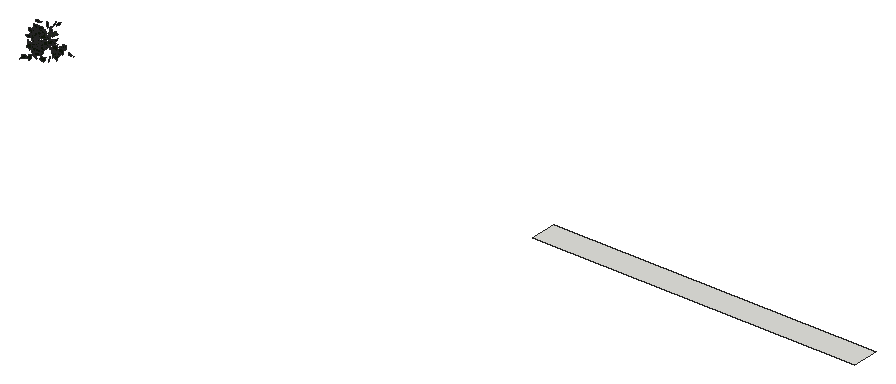
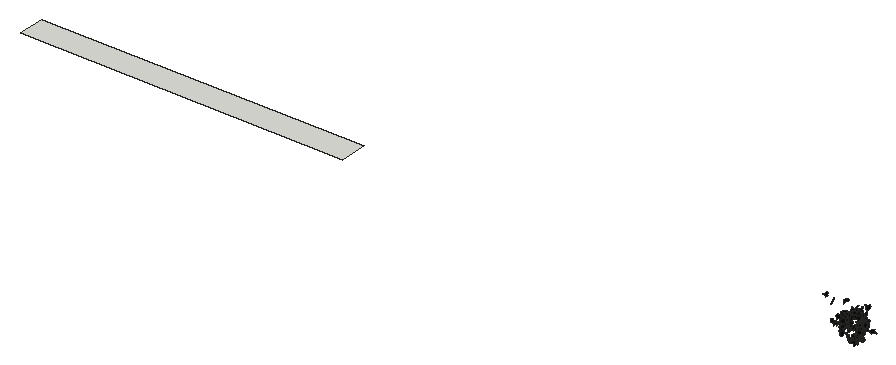
# SketchUp Ruby script. Lengths in inches.
U = 1.inch
M = Sketchup.active_model
def pt(a) = Geom::Point3d.new(a.map { |v| v * U })
def face(e, loops, mat)
  f = e.add_face(loops[0].map { |a| pt(a) })
  loops[1..].each { |l| e.add_face(l.map { |a| pt(a) }).erase! }
  f.material = f.back_material = mat if mat
  f
end
# faces: each face lists its corners as indices into pts; further lists are holes
def faces(e, pts, list, mat = nil) = list.each { |f| face(e, (f[0].is_a?(Array) ? f : [f]).map { |l| l.map { |i| pts[i] } }, mat) }
# xy, xz, yz: faces in a plane at the given z, y or x. An outline is a flat list of corners, or four numbers for a rectangle; further outlines are holes
def ring(l) = l.size == 4 ? [[l[0], l[1]], [l[2], l[1]], [l[2], l[3]], [l[0], l[3]]] : l.each_slice(2).to_a
def flat(e, list, mat, &to3) = list.each { |f| face(e, (f[0].is_a?(Array) ? f : [f]).map { |l| ring(l).map { |u, v| to3.(u, v) } }, mat) }
def xy(e, z, list, mat = nil) = flat(e, list, mat) { |x, y| [x, y, z] }
def xz(e, y, list, mat = nil) = flat(e, list, mat) { |x, z| [x, y, z] }
def yz(e, x, list, mat = nil) = flat(e, list, mat) { |y, z| [x, y, z] }
def lines(e, pts, list) = list.each { |a, b| e.add_line(pt(pts[a]), pt(pts[b])) }
# prism: a flat outline (further loops are holes) pulled along v
def prism(e, loops, v, mat = nil)
  f = face(e, loops, mat); d = Geom::Vector3d.new(v.map { |x| x * U })
  f.pushpull(f.normal.samedirection?(d) ? d.length : -d.length)
end
def box(e, o, s, mat = nil) = prism(e, [[o, [o[0] + s[0], o[1], o[2]], [o[0] + s[0], o[1] + s[1], o[2]], [o[0], o[1] + s[1], o[2]]]], [0, 0, s[2]], mat)
def at(x, y, z, deg = 0) = Geom::Transformation.translation(pt([x, y, z])) * Geom::Transformation.rotation(ORIGIN, Z_AXIS, deg.degrees)
def axes(o, x, y, z) = Geom::Transformation.new([*x, 0, *y, 0, *z, 0, *pt(o).to_a, 1])
def part(name) = M.definitions.add(name)
# library, detail: a bought-in or finely detailed component or shape, given as its bounding box
def library(name, o, s) = part(name).tap { |d| box(d.entities, o, s) }
def detail(e, o, s) = box(e.add_group.entities, o, s)
def put(e, d, t, mat = nil) = e.add_instance(d, t).tap { |i| i.material = mat if mat }
def group(e, t, mat = nil) = e.add_group.tap { |g| g.transformation = t; g.material = mat if mat }.entities
root = M.entities
M.materials.add("efeu1").color = [18, 25, 13]
M.materials.add("efeu2").color = [43, 57, 29]
c1 = part("ivyleaf_10")
p = [[0,0.5,-0.03],[-0.0625,2.02,-0.43],[-0.19,2.01,-0.46],[-0.54,1.05,-0.29],[-0.52,0.625,-0.18],[-0.83,0.76,-0.28],
  [-1.16,0.64,-0.33],[-1.15,0.33,-0.24],[-0.77,-0.39,0.02],[-0.3,-0.51,0.16],[0.04,-0.48,0.23],[-0.02,2.01,-0.4375],
  [-0.06,2.01,-0.43],[0.04,-0.49,0.23],[0.67,-0.49,0.14],[1.38,0.36,-0.2],[1.375,0.51,-0.24],[0.81,0.65,-0.19],
  [0.62,0.59,-0.15],[0.6,1.09,-0.28],[0.5,1.23,-0.31]]
faces(c1.entities,p,[[0,1,2,3,4,5,6,7,8,9,10],[11,12,0,13,14,15,16,17,18,19,20]],"efeu2")
c2 = part("ivyleaf_9")
p = [[1.54,2.16,1.25],[1.36,2.04,1.19],[-0.21,0.99,0.68],[-0.71,1.11,0.82],[-0.85,0.86,0.67],[-0.8,0.17,0.21],
  [-0.9,-0.01,0.1],[-0.67,-0.16,-0.02],[-0.08,-0.08,-0.05],[-0.03,-0.6,-0.4],[0.65,-0.88,-0.66],[0.83,-0.6,-0.49],
  [1.29,-0.42,-0.43],[1.8125,-0.07,-0.26],[1.21,0.44,0.15]]
faces(c2.entities,p,[[0,1,2,3,4,5,6,7,8,9,10,11,12,13,14]],"efeu1")
xy(root,234.35,[[233.9,223.4375,351.16,233.25]])
put(root,c1,axes([53.68,222.76,235.85],[0.26866,-0.3585,-0.22203],[-0.10987,0.19466,-0.44725],[0.40712,0.28911,0.02581]))
put(root,c1,axes([53.39,224.44,234.02],[0.06431,-0.20007,0.45369],[0.33751,-0.31749,-0.18785],[0.36325,0.33041,0.09422]))
put(root,c2,axes([53.25,220.89,238.05],[0.09206,-0.15249,0.4672],[0.48376,-0.05563,-0.11348],[0.08659,0.47292,0.1373]))
put(root,c2,axes([53.3,223.6875,241.74],[0.41396,-0.06275,0.27331],[0.28028,0.10827,-0.39965],[-0.00903,0.48409,0.12482]))
put(root,c2,axes([53.38,223.2,239.45],[0.45441,-0.09026,0.18806],[0.19009,-0.00644,-0.46241],[0.0859,0.49174,0.02846]))
put(root,c2,axes([53.79,222.93,236.93],[0.2925,0.38007,-0.14139],[-0.08119,-0.11592,-0.47955],[-0.39731,0.3035,-0.0061]))
put(root,c1,axes([53.71,222.47,239.98],[0.36999,0.33148,-0.05681],[-0.0427,-0.03749,-0.49676],[-0.33359,0.37245,0.00057]))
put(root,c1,axes([53.66,222.33,238.65],[0.48401,-0.09672,0.07988],[0.0795,-0.00978,-0.49354],[0.09703,0.49046,0.00591]))
put(root,c1,axes([53.44,222.5,240.39],[0.32317,-0.37959,-0.0384],[0.3815,0.32203,0.02744],[0.0039,-0.04703,0.49777]))
put(root,c2,axes([53.7,221.08,240.375],[0.14894,0.13583,0.45757],[0.24086,0.39243,-0.1949],[-0.41207,0.27847,0.05147]))
put(root,c2,axes([53.62,222.21,240.14],[0.24413,-0.42175,-0.11194],[-0.0519,0.0993,-0.48728],[0.43325,0.24954,0.00471]))
put(root,c1,axes([53.51,222.35,241.07],[0.32319,-0.38031,0.03027],[0.38151,0.322,-0.02773],[0.00159,0.04102,0.49831]))
put(root,c2,axes([53.9375,221.61,238.37],[0.22114,-0.11467,-0.43353],[-0.39527,0.17846,-0.24883],[0.2118,0.45277,-0.01173]))
put(root,c1,axes([53.49,221.5625,233.52],[0.06061,-0.08172,0.48954],[0.4629,0.1872,-0.02606],[-0.17902,0.45638,0.09834]))
put(root,c2,axes([53.61,222.13,239.21],[0.48767,-0.1102,-0.00546],[-0.00507,0.00231,-0.49997],[0.11022,0.4877,0.00113]))
put(root,c1,axes([53.97,223.37,234.39],[-0.45789,0.20073,0.00706],[-0.0063,0.0032,-0.49995],[-0.20075,-0.45793,-0.0004]))
put(root,c2,axes([53.83,223.04,237.98],[0.09084,-0.4905,0.03403],[0.00048,-0.03452,-0.49881],[0.49168,0.09065,-0.0058]))
put(root,c2,axes([53.79,220.46,240.29],[0.45416,0.1309,0.16312],[0.15632,0.04662,-0.47264],[-0.13895,0.4803,0.00142]))
put(root,c2,axes([54.3,222.09,237.47],[-0.14055,0.47895,-0.02926],[0.00706,-0.02842,-0.49914],[-0.47979,-0.14072,0.00123]))
put(root,c2,axes([53.87,218.93,236.71],[-0.02657,0.01155,0.49916],[0.20062,-0.45749,0.02126],[0.45722,0.20141,0.01968]))
put(root,c1,axes([54.1,223.16,239.02],[0.49572,-0.06377,-0.01387],[-0.01312,0.00673,-0.49978],[0.06393,0.49587,0.005]))
put(root,c2,axes([54.4375,222.8,239.85],[-0.35492,-0.14761,0.31975],[-0.29035,-0.13428,-0.38427],[0.19932,-0.45845,0.0096]))
put(root,c2,axes([54.45,222.9,239.24],[-0.30345,-0.09684,0.3854],[-0.34664,-0.17261,-0.3163],[0.19431,-0.45916,0.03762]))
put(root,c2,axes([54.48,216.4375,233.95],[-0.04559,0.08062,-0.49135],[-0.06631,-0.48999,-0.07424],[-0.49348,0.05839,0.05536]))
put(root,c2,axes([53.93,221.36,233.76],[0.19913,-0.00962,-0.45854],[0.44578,0.12158,0.19104],[0.10782,-0.4849,0.057]))
put(root,c2,axes([54.51,222.06,239.64],[0.10126,0.48645,-0.05583],[-0.08733,-0.03816,-0.49083],[-0.48179,0.10915,0.07723]))
put(root,c2,axes([54.33,221.63,240.72],[-0.36068,-0.31065,-0.153],[0.18207,0.01779,-0.46533],[0.29456,-0.39138,0.10029]))
put(root,c2,axes([54.17,219.17,236.59],[0.00133,0.00238,-0.49999],[0.49946,-0.02322,0.00122],[-0.02321,-0.49946,-0.00244]))
put(root,c2,axes([54.21,219.32,241.29],[0.25744,-0.4108,0.12233],[0.07922,-0.09464,-0.48453],[0.42125,0.26886,0.01636]))
put(root,c2,axes([54.71,222,240.4],[0.07366,0.47875,0.12397],[-0.04191,0.13093,-0.48073],[-0.49277,0.06043,0.05942]))
put(root,c2,axes([54.68,224.24,234.8125],[-0.21792,-0.23525,0.38363],[-0.18519,-0.3416,-0.31467],[0.41014,-0.27923,0.06175]))
put(root,c2,axes([54.55,221.98,236.875],[0.33559,0.37048,0.01095],[0.00649,0.0089,-0.49988],[-0.37059,0.33565,0.00116]))
put(root,c2,axes([54.79,222.89,234.01],[-0.42098,-0.25223,0.0957],[-0.06874,-0.07121,-0.4901],[0.26087,-0.4258,0.02528]))
put(root,c2,axes([54.25,224.54,233.73],[0.16805,0.0648,-0.46643],[0.42396,0.19476,0.1798],[0.20498,-0.45593,0.01052]))
put(root,c1,axes([54.57,222.51,239.41],[0.19138,0.32142,0.33176],[0.10575,0.31908,-0.37014],[-0.44966,0.21184,0.05415]))
put(root,c2,axes([54.94,222.76,234.95],[-0.17234,0.46328,-0.07533],[0.02638,-0.07056,-0.49429],[-0.46862,-0.17435,-0.00013]))
put(root,c2,axes([54.58,222.29,235.52],[0.09357,-0.49117,0.00023],[-0.00019,-0.00027,-0.5],[0.49117,0.09357,-0.00024]))
put(root,c2,axes([54.55,221.41,241.46],[0.21882,-0.42799,-0.13765],[-0.02779,0.13991,-0.47922],[0.44872,0.21737,0.03744]))
put(root,c2,axes([54.95,220.23,239.47],[0.25303,0.24206,-0.35691],[-0.28127,-0.22104,-0.34932],[-0.32689,0.37756,0.02431]))
put(root,c2,axes([54.55,220.19,235.02],[0.19564,-0.42779,0.16948],[0.07815,-0.15059,-0.47033],[0.45345,0.21052,0.00794]))
put(root,c2,axes([54.71,222.8125,233.62],[0.00939,-0.49768,0.04724],[0.00232,-0.0472,-0.49776],[0.49991,0.00957,0.00142]))
put(root,c2,axes([54.73,222.03,238.28],[-0.00784,-0.49886,0.03276],[0.00334,-0.03282,-0.49891],[0.49993,-0.00761,0.00385]))
put(root,c2,axes([54.84,222.38,234.12],[-0.32946,-0.3441,-0.15184],[0.14826,0.06669,-0.47283],[0.34566,-0.35658,0.05809]))
put(root,c2,axes([54.77,223.11,233.62],[0.43748,0.24204,0.00511],[0.00058,0.00951,-0.49991],[-0.2421,0.43741,0.00804]))
put(root,c1,axes([54.83,222.65,234.34],[0.30397,0.36624,0.1532],[0.02307,0.17634,-0.4673],[-0.39632,0.29116,0.09031]))
put(root,c2,axes([55.1,220.12,238.93],[0.01824,0.2621,-0.4254],[-0.02449,-0.42471,-0.26272],[-0.49907,0.03043,-0.00266]))
put(root,c2,axes([54.83,220.1,234.99],[0.25727,0.24166,0.35413],[0.19377,0.30287,-0.34745],[-0.38244,0.31602,0.06219]))
put(root,c2,axes([55.37,221.4,237.61],[-0.05337,0.05799,0.49375],[-0.45273,0.19949,-0.07237],[-0.20539,-0.4548,0.03122]))
put(root,c2,axes([55.03,220.35,238.73],[0.10845,0.21429,0.43854],[0.11438,0.42557,-0.23623],[-0.47451,0.15156,0.04328]))
put(root,c2,axes([54.89,222.01,239.7],[0.04734,-0.4977,-0.0072],[-0.00899,0.00637,-0.49988],[0.49767,0.04746,-0.00835]))
put(root,c2,axes([54.93,222.37,238.55],[0.02528,-0.4967,-0.05144],[0.05066,0.05379,-0.49451],[0.49678,0.01979,0.05304]))
put(root,c2,axes([55.02,220.33,238.65],[0.46952,0.17189,-0.00156],[-0.00394,0.00621,-0.49995],[-0.17186,0.46948,0.00718]))
put(root,c1,axes([55.2,222.84,233.71],[-0.11722,-0.39959,0.27674],[0.10261,-0.2986,-0.38769],[0.47511,-0.0341,0.15201]))
put(root,c2,axes([55.12,219.08,239.83],[-0.07174,-0.47402,-0.142],[0.03393,0.13843,-0.47926],[0.49366,-0.07839,0.0123]))
put(root,c2,axes([54.97,219.6,234.38],[0.36113,0.09616,0.33218],[0.32276,0.07873,-0.37367],[-0.12417,0.48431,-0.00521]))
put(root,c2,axes([55.33,224.45,234.45],[0.29641,-0.35653,-0.18715],[-0.1052,0.15575,-0.46333],[0.38868,0.31405,0.01732]))
put(root,c2,axes([55.15,219.92,239.17],[0.19663,-0.2263,0.40016],[0.32946,-0.23417,-0.29432],[0.32061,0.37942,0.05702]))
put(root,c2,axes([55.38,223.72,237.98],[0.12631,-0.39172,0.28391],[0.18898,-0.23016,-0.40164],[0.44534,0.20877,0.08991]))
put(root,c2,axes([55.47,222.21,240.66],[-0.00033,-0.07631,-0.49414],[0.12899,0.4774,-0.07381],[0.48307,-0.12753,0.01937]))
put(root,c2,axes([55.95,218.49,237.08],[-0.49985,0.00984,0.0074],[-0.00741,-0.00068,-0.49994],[-0.00983,-0.4999,0.00083]))
put(root,c1,axes([55.82,220.02,237.15],[-0.37967,-0.28779,-0.15174],[-0.11696,-0.09688,0.47638],[-0.30359,0.39723,0.00625]))
put(root,c2,axes([56.02,220.57,239.71],[-0.38356,0.14429,-0.28646],[-0.26941,0.0974,0.4098],[0.17406,0.46871,0.00303]))
put(root,c2,axes([55.69,217.22,237.51],[-0.31252,-0.23213,-0.31377],[0.24241,0.19958,-0.3891],[0.30589,-0.39532,-0.0122]))
put(root,c2,axes([55.64,223.11,235.06],[-0.01153,-0.1965,-0.45962],[0.03085,0.45859,-0.19683],[0.49891,-0.0329,0.00155]))
put(root,c2,axes([55.7,220.07,237.3125],[0.06749,-0.32454,0.37432],[0.05813,-0.36998,-0.33126],[0.492,0.08823,-0.01221]))
put(root,c2,axes([55.69,219.66,241.97],[0.27937,-0.34607,0.22845],[0.1405,-0.18017,-0.44475],[0.39014,0.31269,-0.00342]))
put(root,c2,axes([56.18,220.17,233.23],[0.24474,0.00651,0.43596],[-0.43579,-0.01195,0.24483],[0.0136,-0.49981,-0.00018]))
put(root,c2,axes([55.74,218.89,238.57],[-0.07083,0.0022,-0.49495],[0.49419,0.02813,-0.0706],[0.02753,-0.4992,-0.00616]))
put(root,c2,axes([55.77,218.04,237.05],[0.0278,-0.03365,0.49809],[0.4839,0.1245,-0.01859],[-0.12277,0.48308,0.03948]))
put(root,c2,axes([56.45,216.65,234.02],[-0.39728,0.11069,0.28269],[-0.27067,0.08173,-0.41238],[-0.1375,-0.48069,-0.00502]))
put(root,c2,axes([55.77,216.23,241.06],[0.34931,0.3105,-0.17769],[0.13429,0.11638,0.46736],[0.33158,-0.37423,-0.00209]))
put(root,c1,axes([56.35,224.47,234.27],[-0.15975,-0.31053,0.35785],[-0.16778,-0.31609,-0.34919],[0.44309,-0.23164,-0.00321]))
put(root,c2,axes([56.08,219.97,235.93],[0.07711,-0.43565,-0.23295],[-0.00951,0.23441,-0.44154],[0.49393,0.07252,0.02786]))
put(root,c2,axes([56.07,219.6,239.3],[0.44145,-0.09379,-0.21523],[0.21749,-0.00925,0.45012],[-0.08841,-0.49104,0.03263]))
put(root,c2,axes([56.73,220.11,234.93],[-0.27547,-0.40578,0.09724],[0.06129,0.07591,0.49039],[-0.41275,0.28209,0.00792]))
put(root,c2,axes([56.46,224.88,236.78],[0.28493,-0.35254,-0.21102],[0.13081,-0.1656,0.45328],[-0.38949,-0.31351,-0.00214]))
put(root,c2,axes([56.77,220.03,240.66],[0.30616,0.34876,-0.1861],[-0.13453,-0.12941,-0.46385],[-0.37171,0.3341,0.0146]))
put(root,c2,axes([56.37,218.34,233.88],[0.25138,-0.31975,0.2908],[0.22561,-0.18987,-0.40379],[0.36866,0.33423,0.04882]))
put(root,c2,axes([56.95,218.75,240.5625],[0.19762,0.1217,0.44287],[-0.42378,-0.13756,0.2269],[0.17707,-0.46504,0.04878]))
put(root,c2,axes([57.11,223.65,241.98],[0.11136,-0.01841,-0.48709],[-0.48441,0.05144,-0.11269],[0.05426,0.49701,-0.00638]))
put(root,c2,axes([56.95,221.34,234.03],[-0.42493,-0.04003,-0.26045],[0.2592,0.02549,-0.42681],[0.04745,-0.49774,-0.00092]))
put(root,c1,axes([57.15,224.29,234.84],[0.385,0.04645,0.31562],[-0.31726,0.00378,0.38644],[0.03352,-0.49782,0.03238]))
put(root,c2,axes([56.64,220.68,235.35],[0.17566,-0.03445,-0.46686],[0.43854,0.18657,0.15124],[0.16378,-0.46261,0.09576]))
put(root,c1,axes([57.1,225.05,240.28],[0.35051,-0.32304,0.15095],[0.10899,-0.10448,-0.47666],[0.3395,0.36706,-0.00283]))
put(root,c1,axes([57.36,224.98,238.27],[0.00029,-0.2919,-0.40595],[0.01254,0.40583,-0.2918],[0.49984,-0.01001,0.00756]))
put(root,c1,axes([57.54,224.54,238.75],[0.26519,0.30642,-0.29288],[-0.18784,-0.22475,-0.40522],[-0.37998,0.32496,-0.00409]))
put(root,c2,axes([57.33,225,239.24],[-0.08466,0.01937,-0.4924],[0.41817,-0.2615,-0.08218],[-0.26071,-0.42572,0.02808]))
put(root,c2,axes([57.3,220.71,241.12],[-0.1749,-0.19571,-0.42557],[0.26273,0.33509,-0.26208],[0.38779,-0.3153,-0.01438]))
put(root,c2,axes([57.47,222.43,236.4],[-0.22708,-0.29784,-0.33125],[0.1994,0.26452,-0.37453],[0.39834,-0.3022,-0.00136]))
put(root,c2,axes([57.82,218.53,235.74],[0.30125,-0.15627,0.36719],[-0.32984,0.16146,0.33932],[-0.22462,-0.44667,-0.0058]))
put(root,c2,axes([57.88,222.37,236.05],[0.27422,0.15686,0.38755],[-0.37283,-0.11801,0.31156],[0.18921,-0.45986,0.05224]))
put(root,c2,axes([57.81,225.26,238.3125],[0.02778,0.04806,-0.49691],[-0.13022,0.48115,0.03926],[0.48195,0.12723,0.03925]))
put(root,c2,axes([57.74,219.97,235.71],[-0.16021,-0.36842,-0.29765],[0.13359,0.26631,-0.40154],[0.45441,-0.20819,0.0131]))
put(root,c2,axes([57.625,219.375,240.34],[0.25094,-0.07557,0.42581],[0.40937,-0.11723,-0.26206],[0.13945,0.48015,0.00304]))
put(root,c2,axes([58.25,222.93,236.96],[-0.01304,0.03195,0.49881],[-0.04463,0.49691,-0.03299],[-0.49783,-0.04538,-0.01011]))
put(root,c2,axes([58.45,220.625,241.34],[0.01806,0.0299,-0.49878],[-0.40053,-0.29754,-0.03234],[-0.29874,0.40072,0.0132]))
put(root,c2,axes([57.8125,225.64,235.98],[0.2962,0.378,-0.13923],[0.08236,0.11233,0.48021],[0.39431,-0.3074,0.00428]))
put(root,c2,axes([58.03,218.72,241.61],[0.26873,-0.33607,-0.25465],[-0.09216,0.24785,-0.42435],[0.41145,0.275,0.07127]))
put(root,c2,axes([57.91,216.12,237.48],[0.00237,0.00678,0.49995],[0.38139,-0.32332,0.00257],[0.32333,0.38133,-0.0067]))
put(root,c2,axes([58.01,221.5,240.85],[0.09794,-0.32552,0.36666],[0.13168,-0.34271,-0.33943],[0.4723,0.16305,0.0186]))
put(root,c1,axes([58.07,225.41,238.43],[0.06222,0.15515,0.47123],[0.20317,0.4253,-0.16685],[-0.4526,0.21224,-0.01012]))
put(root,c2,axes([58.39,220.76,239.01],[0.02094,-0.02956,-0.49869],[-0.30956,0.39097,-0.03617],[0.39209,0.31027,-0.00193]))
put(root,c2,axes([58.75,224.8,241.92],[-0.17678,0.43307,0.17664],[-0.07616,0.15966,-0.46766],[-0.46146,-0.19225,0.00952]))
put(root,c2,axes([58.375,220.98,237.49],[0.11682,-0.2661,-0.40687],[-0.08785,0.40001,-0.28684],[0.47816,0.1385,0.0467]))
put(root,c2,axes([59.02,226.03,241.64],[0.13604,0.46658,0.11746],[0.03333,0.11263,-0.48601],[-0.47998,0.14006,-0.00046]))
put(root,c2,axes([59.1,219.06,240.34],[-0.30995,-0.07299,0.3855],[0.37697,0.08075,0.31838],[-0.10874,0.48801,0.00497]))
put(root,c2,axes([59.53,223.66,234.8],[-0.47649,-0.09073,0.12136],[0.11901,0.02377,0.48505],[-0.09379,0.49112,-0.00106]))
put(root,c2,axes([59.55,218.14,233.625],[-0.06703,0.02881,0.49465],[0.4818,-0.11274,0.07186],[0.11567,0.48627,-0.01265]))
put(root,c2,axes([60.1,222.76,235.71],[0.10577,0.37445,0.31401],[0.09064,0.30068,-0.38907],[-0.48021,0.13923,-0.00427]))
put(root,c2,axes([60.0625,217.47,237.65],[0.1506,-0.02151,0.4763],[0.47126,-0.06911,-0.15213],[0.07237,0.49473,-0.00054]))
put(root,c2,axes([60.28,222.19,237.7],[0.40124,-0.02593,0.29721],[0.2973,-0.00679,-0.40195],[0.02489,0.49928,0.00997]))
put(root,c2,axes([60.91,220.0625,239.13],[-0.35201,-0.23977,-0.26192],[0.2247,0.13517,-0.42572],[0.27495,-0.41742,0.0126]))
put(root,c2,axes([61.36,221.89,233.68],[-0.00659,-0.2545,0.43033],[0.03356,0.42917,0.25433],[-0.49883,0.03224,0.01143]))
put(root,c2,axes([61.73,219.83,239.125],[-0.4765,-0.14896,-0.02751],[-0.02181,-0.02239,0.49902],[-0.1499,0.47677,0.01484]))
put(root,c2,axes([61.875,219.5,237.06],[0.25781,-0.23645,0.35725],[0.28326,-0.21872,-0.34918],[0.3214,0.38243,0.02118]))
put(root,c2,axes([62.15,220.64,237.68],[-0.16463,-0.25206,-0.3992],[0.21444,0.33673,-0.30105],[0.42061,-0.27033,-0.00277]))
put(root,c2,axes([62.47,220.17,236.08],[-0.24241,-0.43431,0.05108],[-0.02355,-0.04536,-0.49738],[0.43667,-0.24354,0.00153]))
put(root,c2,axes([62.46,217.68,234.76],[0.0417,0.27029,0.41858],[-0.04965,-0.41569,0.27337],[0.49578,-0.06436,-0.00783]))
put(root,c2,axes([62.84,221.74,235.4],[-0.08252,-0.33172,0.3649],[-0.05097,-0.36226,-0.34084],[0.4905,-0.09345,0.02597]))
put(root,c2,axes([63.04,222.15,236.38],[-0.16677,-0.27392,-0.38361],[0.20118,0.32663,-0.32069],[0.42628,-0.26131,0.00127]))
put(root,c2,axes([63.0625,220.26,235.28],[-0.20682,-0.07328,-0.44928],[0.4453,0.06988,-0.21639],[0.09451,-0.48964,0.03635]))
put(root,c2,axes([63.27,217.09,241.375],[-0.01652,-0.33068,-0.37467],[0.01531,0.37437,-0.33108],[0.49949,-0.02241,-0.00224]))
put(root,c2,axes([64,223,236.89],[-0.28622,0.03953,0.40807],[-0.40242,0.06803,-0.28885],[-0.07835,-0.49377,-0.00713]))
put(root,c2,axes([67.04,218.34,240.6],[0.35658,-0.20713,-0.28275],[-0.23758,0.1537,-0.41222],[0.25769,0.42833,0.01119]))
put(root,c2,axes([70.91,216.41,240.125],[0.34352,-0.15487,0.32864],[0.31172,-0.10667,-0.3761],[0.18661,0.46329,0.02326]))
